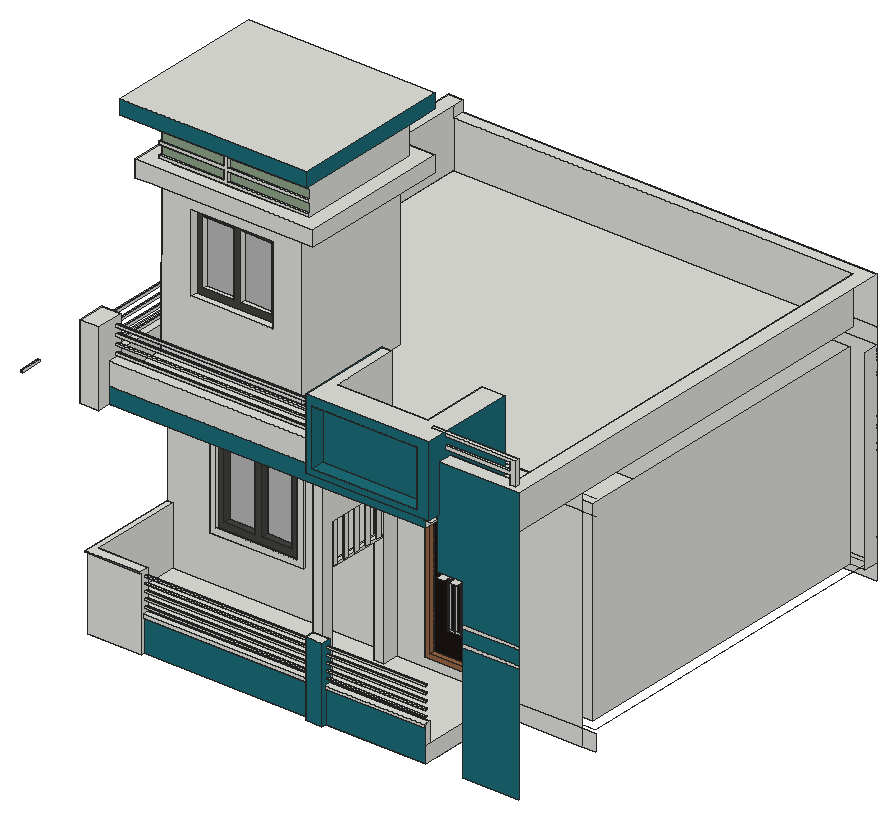
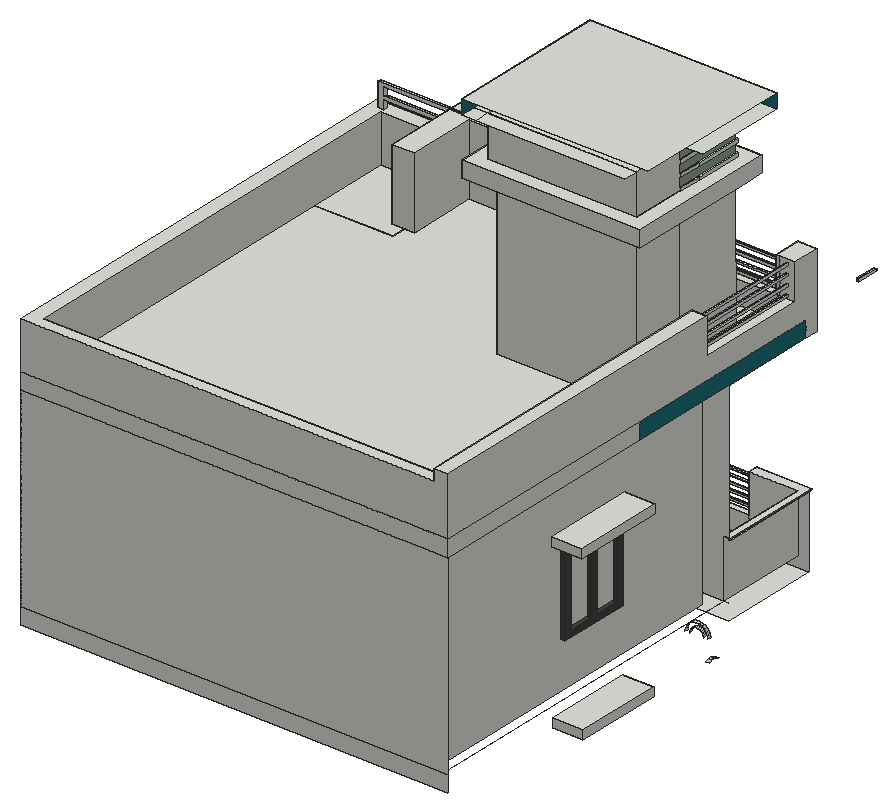
# SketchUp Ruby script. Lengths in inches.
U = 1.inch
M = Sketchup.active_model
def pt(a) = Geom::Point3d.new(a.map { |v| v * U })
def face(e, loops, mat)
  f = e.add_face(loops[0].map { |a| pt(a) })
  loops[1..].each { |l| e.add_face(l.map { |a| pt(a) }).erase! }
  f.material = f.back_material = mat if mat
  f
end
# faces: each face lists its corners as indices into pts; further lists are holes
def faces(e, pts, list, mat = nil) = list.each { |f| face(e, (f[0].is_a?(Array) ? f : [f]).map { |l| l.map { |i| pts[i] } }, mat) }
# xy, xz, yz: faces in a plane at the given z, y or x. An outline is a flat list of corners, or four numbers for a rectangle; further outlines are holes
def ring(l) = l.size == 4 ? [[l[0], l[1]], [l[2], l[1]], [l[2], l[3]], [l[0], l[3]]] : l.each_slice(2).to_a
def flat(e, list, mat, &to3) = list.each { |f| face(e, (f[0].is_a?(Array) ? f : [f]).map { |l| ring(l).map { |u, v| to3.(u, v) } }, mat) }
def xy(e, z, list, mat = nil) = flat(e, list, mat) { |x, y| [x, y, z] }
def xz(e, y, list, mat = nil) = flat(e, list, mat) { |x, z| [x, y, z] }
def yz(e, x, list, mat = nil) = flat(e, list, mat) { |y, z| [x, y, z] }
def lines(e, pts, list) = list.each { |a, b| e.add_line(pt(pts[a]), pt(pts[b])) }
# prism: a flat outline (further loops are holes) pulled along v
def prism(e, loops, v, mat = nil)
  f = face(e, loops, mat); d = Geom::Vector3d.new(v.map { |x| x * U })
  f.pushpull(f.normal.samedirection?(d) ? d.length : -d.length)
end
def box(e, o, s, mat = nil) = prism(e, [[o, [o[0] + s[0], o[1], o[2]], [o[0] + s[0], o[1] + s[1], o[2]], [o[0], o[1] + s[1], o[2]]]], [0, 0, s[2]], mat)
def at(x, y, z, deg = 0) = Geom::Transformation.translation(pt([x, y, z])) * Geom::Transformation.rotation(ORIGIN, Z_AXIS, deg.degrees)
def axes(o, x, y, z) = Geom::Transformation.new([*x, 0, *y, 0, *z, 0, *pt(o).to_a, 1])
def part(name) = M.definitions.add(name)
# library, detail: a bought-in or finely detailed component or shape, given as its bounding box
def library(name, o, s) = part(name).tap { |d| box(d.entities, o, s) }
def detail(e, o, s) = box(e.add_group.entities, o, s)
def put(e, d, t, mat = nil) = e.add_instance(d, t).tap { |i| i.material = mat if mat }
def group(e, t, mat = nil) = e.add_group.tap { |g| g.transformation = t; g.material = mat if mat }.entities
root = M.entities
M.materials.add("Glass_Mirror_01").color = [185, 185, 185]
M.materials.add("I06_Sapphire_Night").color = [28, 110, 122]
M.materials.add("M04_Stone_Frost").color = [142, 163, 138]
M.materials.add("M05_Graphite_Haze").color = [114, 114, 114]
M.materials.add("Wood_Floor_12_1K").color = [28, 22, 19]
M.materials.add("Wood_Planks_01_1K").color = [69, 67, 63]
M.materials.add("Wood_Veneer_15_1K").color = [153, 102, 66]
box(root,[5.27,10.71,299.4],[1.43,13.32,1.36])
xy(root,139.3,[[15.64,197.5,18.64,213.54],[15.64,217.54,18.64,233.59]],"Wood_Planks_01_1K")
xy(root,143.3,[[15.64,193.5,18.64,237.59]])
xy(root,144,[[153.64,45,153.64,48,51.78,48,51.78,46,18.64,46,18.64,108,153.64,108,153.64,50.875,159.64,50.875,159.64,56.88,225.64,56.88,225.64,108,225.72,108,225.72,48,164.1,48,164.1,45],[153.64,50.875,153.64,108,225.64,108,225.64,56.88,159.64,56.88,159.64,50.875],[153.64,50.875,159.64,108],[159.64,56.88,225.64,108]])
xy(root,144.51,[[0,189.1,18.64,243.39]])
xy(root,149.79,[[0,189.1,18.64,243.39]])
xy(root,154,[[225.64,48,225.72,48,225.72,108,159.64,108,159.64,98,153.64,98,153.64,108,21.64,108,21.64,51,153.64,51,153.64,58,159.64,58,159.64,51,225.64,51],[153.64,50.875,159.64,51],[153.64,51,159.64,58],[27.64,117,273.64,315]])
xy(root,160,[[177.64,108,213.64,117]])
xy(root,160,[[177.64,107,213.64,108]],"Wood_Veneer_15_1K")
xy(root,163,[[180.64,110.5,210.64,117]])
xy(root,163,[[180.64,107,210.64,110.5]],"Wood_Veneer_15_1K")
xy(root,164,[[51.78,47,153.64,48],[164.1,47,225.64,48]])
xy(root,166,[[51.78,47,153.64,47,153.64,50.875,164.1,50.875,164.1,47,225.64,47,225.64,51,51.78,51]])
xy(root,169.1,[[51.78,47.89,225.64,49.04]])
xy(root,170.1,[[51.78,47.89,225.64,49.04]])
xy(root,173.43,[[51.78,47.89,225.64,49.04]])
xy(root,174.42,[[51.78,47.89,225.64,49.04]])
xy(root,177.74,[[190.19,109.5,202.59,110.5]])
xy(root,177.75,[[51.78,47.89,225.64,49.04]])
xy(root,178.74,[[51.78,47.89,225.64,49.04],[191.19,109.5,193.99,110.5],[194.99,109.5,197.79,110.5],[198.79,109.5,201.59,110.5]])
xy(root,182.08,[[51.78,47.89,225.64,49.04]])
xy(root,182.6,[[45.44,106.82,103.01,108]])
xy(root,183.07,[[51.78,47.89,225.64,49.04]])
xy(root,186.4,[[51.78,47.89,225.64,49.04],[49.24,106.82,99.21,108]])
xy(root,187.39,[[51.78,47.89,225.64,49.04]])
xy(root,189,[[17.64,45,50.78,46],[50.78,45,51.78,46],[17.64,46,18.64,107],[17.64,107,18.64,108]])
xy(root,190,[[17.64,45,51.78,45,51.78,51,21.64,51,21.64,108,17.64,108],[153.64,45,164.1,50.875]])
xy(root,190.4,[[53.24,112.5,72.22,117],[76.22,112.5,95.21,117]])
xy(root,190.4,[[53.24,108,72.22,112.5],[76.22,108,95.21,112.5]],"Wood_Planks_01_1K")
xy(root,190.875,[[15.64,193.5,18.64,237.59]],"Wood_Planks_01_1K")
xy(root,194.875,[[15.64,197.5,18.64,213.54],[15.64,217.54,18.64,233.59]],"Wood_Planks_01_1K")
xy(root,205.66,[[191.19,109.5,193.99,110.5],[194.99,109.5,197.79,110.5],[198.79,109.5,201.59,110.5]])
xy(root,206.43,[[191.19,109.5,193.99,110.5],[194.99,109.5,197.79,110.5],[198.79,109.5,201.59,110.5]])
xy(root,223.3125,[[155.41,58,158.36,98]])
xy(root,224.34,[[191.19,109.5,193.99,110.5],[194.99,109.5,197.79,110.5],[198.79,109.5,201.59,110.5]])
xy(root,224.66,[[155.41,58,158.36,58,158.36,59.95,158.14,59.95,158.14,62.61,158.36,62.61,158.36,68.33,158.14,68.33,158.14,70.98,158.36,70.98,158.36,76.7,158.14,76.7,158.14,79.36,158.36,79.36,158.36,85.08,158.14,85.08,158.14,87.73,158.36,87.73,158.36,93.45,158.14,93.45,158.14,96.11,158.36,96.11,158.36,98,155.41,98],[158.14,59.95,158.36,62.61],[158.36,59.95,159.05,62.61],[158.14,68.33,158.36,70.98],[158.36,68.33,159.05,70.98],
  [158.14,76.7,158.36,79.36],[158.36,76.7,159.05,79.36],[158.14,85.08,158.36,87.73],[158.36,85.08,159.05,87.73],[158.14,93.45,158.36,96.11],
  [158.36,93.45,159.05,96.11]])
xy(root,225.34,[[190.19,109.5,202.59,110.5]])
xy(root,237.72,[[53.24,112.5,72.22,117],[76.22,112.5,95.21,117]])
xy(root,237.72,[[53.24,108,72.22,112.5],[76.22,108,95.21,112.5]],"Wood_Planks_01_1K")
xy(root,237.76,[[15.64,197.5,18.64,213.54],[15.64,217.54,18.64,233.59]],"Wood_Planks_01_1K")
xy(root,241,[[180.64,110.5,210.64,117]])
xy(root,241,[[180.64,107,210.64,110.5]],"Wood_Veneer_15_1K")
xy(root,241.72,[[49.24,106.82,99.21,108]])
xy(root,241.76,[[15.64,193.5,18.64,237.59]],"Wood_Planks_01_1K")
xy(root,244,[[177.64,108,213.64,117]])
xy(root,244,[[177.64,107,213.64,108]],"Wood_Veneer_15_1K")
xy(root,244.92,[[0,187.98,18.64,244.27]])
xy(root,245.52,[[45.44,106.82,103.01,108]])
xy(root,250,[[[153.64,58,159.64,98],[158.14,85.08,159.05,87.73],[158.14,76.7,159.05,79.36],[158.14,68.33,159.05,70.98],[158.14,59.95,159.05,62.61],[158.14,93.45,159.05,96.11]],[158.14,59.95,159.05,62.61],[158.14,68.33,159.05,70.98],[158.14,76.7,159.05,79.36],[158.14,85.08,159.05,87.73],
  [158.14,93.45,159.05,96.11]])
xy(root,250.47,[[0,187.98,18.64,244.27]])
xy(root,252.41,[[236.45,43,240.8,48],[244.33,43,248.68,48]])
xy(root,274,[[18.64,40,30.27,48],[18.64,48,18.64,108,153.64,108,153.64,50.875,159.64,50.875,159.64,108,225.72,108,225.72,48]])
xy(root,281.97,[[228.57,43,232.92,48]])
xy(root,284,[[18.64,48,225.72,48,225.72,57,225.64,57,225.64,108,273.64,108,273.64,317.1,27.64,317.1,27.64,324,18.64,324],[225.64,57,225.72,108],[225.72,57,273.64,108]])
xy(root,284.16,[[18.64,48,18.64,324,27.64,324,27.64,57,157.87,57,157.87,98.875,163.87,98.875,163.87,57,219.64,57,219.64,98.875,233.62,98.875,233.62,57,225.64,57,225.64,48]])
xy(root,284.16,[[157.87,40,233.62,48]],"I06_Sapphire_Night")
xy(root,288.16,[[161.87,40,226.3,48]],"I06_Sapphire_Night")
xy(root,298.07,[[30.27,48,157.87,57],[18.64,57,27.64,124.99]])
xy(root,299.02,[[22.93,57,24.36,121.44],[22.93,121.44,24.36,124.99]])
xy(root,299.4,[[30.27,52.5,157.87,53.93]])
xy(root,300.38,[[22.93,57,24.36,121.44],[22.93,121.44,24.36,124.99]])
xy(root,300.76,[[30.27,52.5,157.87,53.93]])
xy(root,304.59,[[30.27,52.5,157.87,53.93]])
xy(root,304.82,[[22.93,57,24.36,121.44],[22.93,121.44,24.36,124.99]])
xy(root,305.95,[[30.27,52.5,157.87,53.93]])
xy(root,306.18,[[22.93,57,24.36,121.44],[22.93,121.44,24.36,124.99]])
xy(root,309.78,[[30.27,52.5,157.87,53.93]])
xy(root,310.63,[[22.93,57,24.36,121.44],[22.93,121.44,24.36,124.99]])
xy(root,311.14,[[30.27,52.5,157.87,53.93]])
xy(root,311.99,[[22.93,57,24.36,121.44],[22.93,121.44,24.36,124.99]])
xy(root,313.32,[[[233.62,48,282.64,48,282.64,324,27.64,324,27.64,317.1,273.64,317.1,273.64,57,233.62,57],[274.2,52.33,277.71,54.32]],[225.64,48,233.62,57]])
xy(root,314.97,[[30.27,52.5,157.87,53.93]])
xy(root,316.33,[[30.27,52.5,157.87,53.93]])
xy(root,316.43,[[22.93,57,24.36,121.44],[22.93,121.44,24.36,124.99]])
xy(root,317.79,[[22.93,57,24.36,121.44],[22.93,121.44,24.36,124.99]])
xy(root,318.66,[[225.69,52.33,274.2,54.32]])
xy(root,320,[[18.64,40,30.27,57],[18.64,124.99,27.64,324]])
xy(root,320.03,[[45.8,91.34,96.39,95.875]])
xy(root,320.71,[[225.69,52.33,274.2,54.32]])
xy(root,322.89,[[161.87,40,226.3,48]])
xy(root,324.03,[[49.8,95.875,69.1,98.875],[73.1,95.875,92.39,98.875]])
xy(root,325.78,[[225.69,52.33,274.2,54.32]])
xy(root,327.87,[[157.87,40,233.62,40,233.62,52.33,225.69,52.33,225.69,54.32,233.62,54.32,233.62,98.875,219.64,98.875,219.64,57,163.87,57,163.87,98.875,157.87,98.875],[225.69,52.33,233.62,54.32],[233.62,52.33,277.71,54.32]])
xy(root,364.13,[[49.8,95.875,69.1,98.875],[73.1,95.875,92.39,98.875]])
xy(root,368.13,[[45.8,91.34,96.39,95.875]])
xy(root,380.13,[[27.82,82.27,114.51,91.34],[27.82,91.34,114.51,167.15],[27.82,167.15,114.51,176.22]])
xy(root,390.13,[[27.84,90.34,67.09,91.34],[67.09,90.34,69.71,91.34],[69.71,90.34,119.53,91.34],[26.84,120.18,27.84,134.17]])
xy(root,392.13,[[26.84,90.34,27.84,120.18],[27.84,90.34,67.09,91.34],[69.71,90.34,119.53,91.34],[26.84,120.18,27.84,134.17]])
xy(root,397.81,[[26.85,90.34,27.85,120.18],[27.85,90.34,67.1,91.34],[69.72,90.34,119.54,91.34],[26.85,120.18,27.85,134.17]])
xy(root,399.81,[[26.86,90.34,27.86,120.18],[27.86,90.34,67.1,91.34],[69.72,90.34,119.55,91.34],[26.86,120.18,27.86,134.17]])
xy(root,405.49,[[26.87,90.34,27.87,120.18],[27.87,90.34,67.12,91.34],[69.73,90.34,119.56,91.34],[26.87,120.18,27.87,134.17]])
xy(root,407.49,[[26.875,90.34,27.875,120.18],[27.875,90.34,67.12,91.34],[69.74,90.34,119.56,91.34],[26.875,120.18,27.875,134.17]])
xy(root,413.16,[[27.88,90.34,67.13,91.34],[69.75,90.34,119.57,91.34]])
xy(root,415.16,[[27.89,77.1875,119.58,90.34],[27.89,90.34,119.58,167.15],[27.89,167.15,119.58,176.1875]])
xz(root,40,[[18.64,274,30.27,320]])
xz(root,40,[[[157.87,284.16,233.62,327.87],[161.87,288.16,226.3,322.89]]],"I06_Sapphire_Night")
xz(root,45,[[153.64,144,164.1,190]],"I06_Sapphire_Night")
xz(root,45,[[17.64,189,51.78,190]],"M05_Graphite_Haze")
xz(root,46,[[18.64,144,51.78,189]])
xz(root,47,[[51.78,164,153.64,166],[164.1,164,225.64,166]])
xz(root,47.89,[[51.78,169.1,225.64,170.1],[51.78,173.43,225.64,174.42],[51.78,177.75,225.64,178.74],[51.78,182.08,225.64,183.07],[51.78,186.4,225.64,187.39]])
xz(root,48,[[225.64,144,225.72,154],[248.68,216.18,282.64,218.18],[248.68,226.69,282.64,228.69],[18.64,274,30.27,284],[225.64,274,225.72,284],
  [18.64,284,30.27,284.16],[157.87,284,225.64,284.16],[225.64,284,225.72,284,232.92,284.15,232.92,284.16,225.64,284.16],[232.92,284.15,233.62,284.16,232.92,284.16],[30.27,284.16,157.87,298.07],
  [225.64,284.16,233.62,284.16,233.62,313.32,226.3,313.32,226.3,288.16,225.64,288.16]])
xz(root,48,[[51.78,144,153.64,164],[164.1,144,225.64,164],[248.68,144,282.64,216.18],[248.68,218.18,282.64,226.69],[248.68,228.69,282.64,228.69,282.64,313.32,233.62,313.32,233.62,284.16,232.92,284.15,232.92,252.41,248.68,252.41],
  [30.27,274,225.64,284],[161.87,288.16,226.3,322.89]],"I06_Sapphire_Night")
xz(root,49.04,[[51.78,169.1,225.64,170.1],[51.78,173.43,225.64,174.42],[51.78,177.75,225.64,178.74],[51.78,182.08,225.64,183.07],[51.78,186.4,225.64,187.39]])
xz(root,50.875,[[153.64,154,159.64,166],[153.64,166,159.64,190],[159.64,166,164.1,190],[153.64,190,159.64,274]])
xz(root,51,[[21.64,154,51.78,190],[51.78,154,225.64,166]])
xz(root,52.33,[[274.2,313.32,277.71,313.32,277.71,327.87,225.69,327.87,225.69,325.78,274.2,325.78,274.2,320.71,225.69,320.71,225.69,318.66,274.2,318.66]])
xz(root,52.5,[[30.27,299.4,157.87,300.76],[30.27,304.59,157.87,305.95],[30.27,309.78,157.87,311.14],[30.27,314.97,157.87,316.33]])
xz(root,53.93,[[30.27,299.4,157.87,300.76],[30.27,304.59,157.87,305.95],[30.27,309.78,157.87,311.14],[30.27,314.97,157.87,316.33]])
xz(root,54.32,[[274.2,313.32,274.2,318.66,225.69,318.66,225.69,320.71,274.2,320.71,274.2,325.78,225.69,325.78,225.69,327.87,277.71,327.87,277.71,313.32]])
xz(root,57,[[225.64,284,225.64,284.16,233.62,284.16,233.62,313.32,273.64,313.32,273.64,284],[27.64,284.16,157.87,298.07],[163.87,284.16,219.64,327.87],[225.64,284.16,233.62,313.32],[[18.64,298.07,27.64,320],[22.93,316.43,24.36,317.79],[22.93,304.82,24.36,306.18],[22.93,299.02,24.36,300.38],[22.93,310.63,24.36,311.99]],
  [27.64,298.07,30.27,320]])
xz(root,58,[[[153.64,154,159.64,250],[155.41,223.3125,158.36,224.66]],[155.41,223.3125,158.36,224.66]])
xz(root,59.95,[[158.14,224.66,159.05,250]])
xz(root,62.61,[[158.14,224.66,159.05,250]])
xz(root,68.33,[[158.14,224.66,159.05,250]])
xz(root,70.98,[[158.14,224.66,159.05,250]])
xz(root,76.7,[[158.14,224.66,159.05,250]])
xz(root,77.1875,[[128.58,415.15,128.6,423.97,13.75,424.19,13.74,415.19,27.89,415.16,119.58,415.16]],"I06_Sapphire_Night")
xz(root,79.36,[[158.14,224.66,159.05,250]])
xz(root,82.27,[[128.58,380.1,128.59,389.9375,18.77,390.15,18.75,380.15,27.82,380.13,114.51,380.13]])
xz(root,85.08,[[158.14,224.66,159.05,250]])
xz(root,87.73,[[158.14,224.66,159.05,250]])
xz(root,90.34,[[26.84,390.13,119.53,390.13,119.53,392.13,69.71,392.13,69.72,397.81,119.54,397.81,119.55,399.81,69.72,399.81,69.73,405.49,119.56,405.49,119.56,407.49,69.74,407.49,69.75,413.16,119.57,413.16,119.58,415.16,27.89,415.16,26.89,415.17,26.88,413.17,27.88,413.16,67.13,413.16,67.12,407.49,26.875,407.49,26.87,405.49,67.12,405.49,67.1,399.81,26.86,399.81,26.85,397.81,67.1,397.81,67.09,392.13,26.84,392.13]])
xz(root,91.34,[[[114.33,284,114.51,380.13,27.82,380.13,27.64,284.36,27.64,284.16],[45.8,320.03,96.39,368.13]],[119.53,389.96,119.53,390.13,69.71,390.13,69.71,390.05,114.53,389.97],[69.71,390.05,69.71,390.13,67.09,390.13,67.09,390.06],[67.09,390.06,67.09,390.13,27.84,390.13]])
xz(root,91.34,[[27.84,392.13,67.09,392.13,67.1,397.81,27.85,397.81],[69.71,392.13,119.53,392.13,119.54,397.81,69.72,397.81],[27.86,399.81,67.1,399.81,67.12,405.49,27.87,405.49],[69.72,399.81,119.55,399.81,119.56,405.49,69.73,405.49],[27.875,407.49,67.12,407.49,67.13,413.16,27.88,413.16,27.88,411.16],
  [69.74,407.49,119.56,407.49,119.57,413.16,69.75,413.16]],"M04_Stone_Frost")
xz(root,93.45,[[158.14,224.66,159.05,250]])
xz(root,95.875,[[[45.8,320.03,96.39,368.13],[49.8,324.03,69.1,364.13],[73.1,324.03,92.39,364.13]]],"Wood_Planks_01_1K")
xz(root,96.11,[[158.14,224.66,159.05,250]])
xz(root,98,[[[153.64,154,159.64,250],[155.41,223.3125,158.36,224.66]],[155.41,223.3125,158.36,224.66]])
xz(root,98.875,[[157.87,284.16,163.87,327.87],[219.64,284.16,233.62,327.87]])
xz(root,98.875,[[49.8,324.03,69.1,364.13],[73.1,324.03,92.39,364.13]],"Glass_Mirror_01")
xz(root,106.82,[[[45.44,182.6,103.01,245.52],[49.24,186.4,99.21,241.72]]])
xz(root,107,[[[177.64,160,213.64,244],[180.64,163,210.64,241]]],"Wood_Veneer_15_1K")
xz(root,108,[[225.64,144,225.72,154],[225.72,144,231.64,154],[231.64,144,273.64,154],[273.64,144,282.64,154],[[21.64,154,153.64,154,153.64,274,18.64,274,18.64,190,21.64,190],[45.44,182.6,103.01,245.52]],
  [[159.64,154,225.64,274],[177.64,160,213.64,244]],[225.64,154,231.64,274],[231.64,154,273.64,274],[225.64,274,225.72,284],[225.72,274,231.64,284],
  [231.64,274,273.64,284]])
xz(root,108,[[17.64,189,18.64,190]],"M05_Graphite_Haze")
xz(root,108,[[[49.24,186.4,99.21,241.72],[53.24,190.4,72.22,237.72],[76.22,190.4,95.21,237.72]]],"Wood_Planks_01_1K")
xz(root,109.5,[[[190.19,177.74,202.59,225.34],[198.79,178.74,198.79,205.66,201.59,205.66,201.59,206.43,198.79,206.43,198.79,224.34,201.59,224.34,201.59,178.74],[194.99,178.74,197.79,205.66],[191.19,178.74,193.99,205.66],[194.99,206.43,197.79,224.34],[191.19,206.43,193.99,224.34]]])
xz(root,110.5,[[[180.64,163,210.64,241],[190.19,177.74,202.59,225.34]],[191.19,178.74,193.99,205.66],[194.99,178.74,197.79,205.66],[198.79,178.74,201.59,205.66],[191.19,206.43,193.99,224.34],
  [194.99,206.43,197.79,224.34],[198.79,206.43,201.59,224.34]],"Wood_Floor_12_1K")
xz(root,112.5,[[53.24,190.4,72.22,237.72],[76.22,190.4,95.21,237.72]],"Glass_Mirror_01")
xz(root,117,[[[27.64,154,273.64,274],[177.64,160,213.64,244],[53.24,190.4,72.22,237.72],[76.22,190.4,95.21,237.72]]])
xz(root,120.18,[[26.84,390.13,27.84,392.13],[26.85,397.81,27.85,397.81,27.86,399.81,26.86,399.81],[26.87,405.49,27.87,405.49,27.875,407.49,26.875,407.49],[27.88,413.16,27.89,415.16,26.89,415.17,26.88,413.17]])
xz(root,121.44,[[22.93,299.02,24.36,300.38],[22.93,304.82,24.36,306.18],[22.93,310.63,24.36,311.99],[22.93,316.43,24.36,317.79]])
xz(root,124.99,[[[18.64,298.07,27.64,320],[22.93,299.02,24.36,300.38],[22.93,304.82,24.36,306.18],[22.93,310.63,24.36,311.99],[22.93,316.43,24.36,317.79]]])
xz(root,157.4,[[177.64,160,213.64,244]])
xz(root,167.15,[[114.33,284,27.64,284.16,27.64,284.36,27.82,380.13,114.51,380.13],[119.53,389.96,27.84,390.13,27.89,415.16,119.58,415.16]])
xz(root,176.22,[[128.58,380.1,114.51,380.13,27.82,380.13,18.75,380.15,18.77,390.15,27.84,390.13,128.59,389.9375]])
xz(root,187.98,[[0,244.92,18.64,250.47]])
xz(root,189.1,[[0,144.51,18.64,149.79]])
xz(root,193.5,[[15.64,190.875,18.64,241.76]])
xz(root,197.5,[[15.64,194.875,18.64,237.76]],"Wood_Planks_01_1K")
xz(root,213.54,[[15.64,194.875,18.64,237.76]])
xz(root,217.54,[[15.64,194.875,18.64,237.76]],"Wood_Planks_01_1K")
xz(root,233.59,[[15.64,194.875,18.64,237.76]])
xz(root,237.59,[[15.64,190.875,18.64,241.76]],"Wood_Planks_01_1K")
xz(root,243.39,[[0,144.51,18.64,149.79]])
xz(root,244.27,[[0,244.92,18.64,250.47]])
xz(root,315,[[27.64,154,273.64,274]])
xz(root,317.1,[[27.64,284,273.64,313.32]])
xz(root,324,[[18.64,144,282.64,154],[18.64,154,282.64,274],[18.64,274,282.64,284],[27.64,284,27.64,284.16,18.64,284.16,18.64,320,27.64,320,27.64,313.32,282.64,313.32,282.64,284]])
yz(root,0,[[189.1,144.51,243.39,149.79],[187.98,244.92,244.27,250.47]])
yz(root,15.64,[[[193.5,190.875,237.59,241.76],[217.54,194.875,233.59,237.76],[197.5,194.875,213.54,237.76]]],"Wood_Planks_01_1K")
yz(root,17.64,[[45,189,108,190]],"M05_Graphite_Haze")
yz(root,18.64,[[197.5,194.875,213.54,237.76],[217.54,194.875,233.59,237.76],[40,274,40,320,57,320,57,298.07,124.99,298.07,124.99,320,324,320,324,284.16,48,284.16,48,274],[176.54,274,324,284]])
yz(root,18.64,[[48,274,176.54,284]],"I06_Sapphire_Night")
yz(root,21.64,[[51,154,108,190]])
yz(root,22.93,[[57,299.02,121.44,300.38],[121.44,299.02,124.99,300.38],[57,304.82,121.44,306.18],[121.44,304.82,124.99,306.18],[57,310.63,121.44,311.99],
  [121.44,310.63,124.99,311.99],[57,316.43,121.44,317.79],[121.44,316.43,124.99,317.79]])
yz(root,24.36,[[57,299.02,121.44,300.38],[121.44,299.02,124.99,300.38],[57,304.82,121.44,306.18],[121.44,304.82,124.99,306.18],[57,310.63,121.44,311.99],
  [121.44,310.63,124.99,311.99],[57,316.43,121.44,317.79],[121.44,316.43,124.99,317.79]])
yz(root,26.84,[[90.34,390.13,120.18,392.13],[120.18,390.13,134.17,392.13]])
yz(root,27.64,[[117,154,315,274],[317.1,284,324,284.16],[57,284.16,91.34,284.16,91.34,284.36,167.15,284.36,167.15,284.16,317.1,284.16,317.1,320,124.99,320,124.99,298.07,57,298.07],[91.34,284.16,134.17,284.36],[134.17,284.16,167.15,284.36],
  [134.17,284.16,167.15,284.36],[317.1,313.32,324,320]])
yz(root,30.27,[[[40,274,48,274,48,298.07,57,298.07,57,320,40,320],[52.5,314.97,53.93,316.33],[52.5,309.78,53.93,311.14],[52.5,304.59,53.93,305.95],[52.5,299.4,53.93,300.76]]])
yz(root,45.44,[[106.82,182.6,108,245.52]])
yz(root,45.8,[[91.34,320.03,95.875,368.13]])
yz(root,49.24,[[106.82,186.4,108,241.72]])
yz(root,49.8,[[95.875,324.03,98.875,364.13]])
yz(root,51.78,[[[46,144,46,189,45,189,45,190,51,190,51,166,47,166,47,164,48,164,48,144],[47.89,186.4,49.04,187.39],[47.89,182.08,49.04,183.07],[47.89,177.75,49.04,178.74],[47.89,173.43,49.04,174.42],[47.89,169.1,49.04,170.1]],[47.89,169.1,49.04,170.1],[47.89,173.43,49.04,174.42],[47.89,177.75,49.04,178.74],[47.89,182.08,49.04,183.07],
  [47.89,186.4,49.04,187.39]])
yz(root,53.24,[[112.5,190.4,117,237.72]])
yz(root,53.24,[[108,190.4,112.5,237.72]],"Wood_Planks_01_1K")
yz(root,69.1,[[95.875,324.03,98.875,364.13]])
yz(root,72.22,[[112.5,190.4,117,237.72]])
yz(root,72.22,[[108,190.4,112.5,237.72]],"Wood_Planks_01_1K")
yz(root,73.1,[[95.875,324.03,98.875,364.13]])
yz(root,76.22,[[112.5,190.4,117,237.72]])
yz(root,76.22,[[108,190.4,112.5,237.72]],"Wood_Planks_01_1K")
yz(root,92.39,[[95.875,324.03,98.875,364.13]])
yz(root,95.21,[[112.5,190.4,117,237.72]])
yz(root,95.21,[[108,190.4,112.5,237.72]],"Wood_Planks_01_1K")
yz(root,96.39,[[91.34,320.03,95.875,368.13]])
yz(root,99.21,[[106.82,186.4,108,241.72]])
yz(root,103.01,[[106.82,182.6,108,245.52]])
yz(root,153.64,[[50.875,154,50.875,274,108,274,108,154,98,154,98,250,58,250,58,154]])
yz(root,153.64,[[45,144,45,190,50.875,190,50.875,166,47,166,47,164,48,164,48,144]],"I06_Sapphire_Night")
yz(root,155.41,[[58,223.3125,98,224.66]])
yz(root,157.87,[[[40,284.16,40,327.87,98.875,327.87,98.875,284.16,57,284.16,57,298.07,48,298.07,48,284.16],[52.5,314.97,53.93,316.33],[52.5,309.78,53.93,311.14],[52.5,304.59,53.93,305.95],[52.5,299.4,53.93,300.76]]],"I06_Sapphire_Night")
yz(root,158.14,[[59.95,224.66,62.61,250],[68.33,224.66,70.98,250],[76.7,224.66,79.36,250],[85.08,224.66,87.73,250],[93.45,224.66,96.11,250]])
yz(root,158.36,[[58,223.3125,98,224.66]])
yz(root,159.05,[[59.95,224.66,62.61,250],[68.33,224.66,70.98,250],[76.7,224.66,79.36,250],[85.08,224.66,87.73,250],[93.45,224.66,96.11,250]])
yz(root,159.64,[[50.875,154,58,154,58,250,98,250,98,154,108,154,108,274,50.875,274]])
yz(root,161.87,[[40,288.16,48,322.89]],"I06_Sapphire_Night")
yz(root,163.87,[[57,284.16,98.875,327.87]])
yz(root,164.1,[[45,144,48,144,48,164,47,164,47,166,50.875,166,50.875,190,45,190]],"I06_Sapphire_Night")
yz(root,177.64,[[108,160,117,244]])
yz(root,177.64,[[107,160,108,244]],"Wood_Veneer_15_1K")
yz(root,180.64,[[110.5,163,117,241]])
yz(root,180.64,[[107,163,110.5,241]],"Wood_Veneer_15_1K")
yz(root,190.19,[[109.5,177.74,110.5,225.34]])
yz(root,191.19,[[109.5,178.74,110.5,205.66],[109.5,206.43,110.5,224.34]])
yz(root,193.99,[[109.5,178.74,110.5,205.66],[109.5,206.43,110.5,224.34]])
yz(root,194.99,[[109.5,178.74,110.5,205.66],[109.5,206.43,110.5,224.34]])
yz(root,197.79,[[109.5,178.74,110.5,205.66],[109.5,206.43,110.5,224.34]])
yz(root,198.79,[[109.5,178.74,110.5,205.66],[109.5,206.43,110.5,224.34]])
yz(root,201.59,[[109.5,178.74,110.5,205.66],[109.5,205.66,110.5,206.43],[109.5,206.43,110.5,224.34]])
yz(root,202.59,[[109.5,177.74,110.5,178.74],[109.5,178.74,110.5,224.34],[109.5,224.34,110.5,225.34]])
yz(root,210.64,[[110.5,163,117,241]])
yz(root,210.64,[[107,163,110.5,241]],"Wood_Veneer_15_1K")
yz(root,213.64,[[108,160,117,244]])
yz(root,213.64,[[107,160,108,244]],"Wood_Veneer_15_1K")
yz(root,219.64,[[57,284.16,98.875,327.87]])
yz(root,225.64,[[48,154,51,166],[47,164,48,166],[47.89,169.1,48,170.1],[48,169.1,49.04,170.1],[47.89,173.43,48,174.42],
  [48,173.43,49.04,174.42],[47.89,177.75,48,178.74],[48,177.75,49.04,178.74],[47.89,182.08,48,183.07],[48,182.08,49.04,183.07],
  [47.89,186.4,48,187.39],[48,186.4,49.04,187.39]])
yz(root,225.69,[[52.33,318.66,54.32,320.71],[52.33,325.78,54.32,327.87]])
yz(root,225.72,[[48,144,108,154],[48,274,108,284]])
yz(root,226.3,[[40,288.16,48,322.89]],"I06_Sapphire_Night")
yz(root,233.62,[[40,284.16,48,284.16,48,313.32,57,313.32,57,284.16,98.875,284.16,98.875,327.87,40,327.87]],"I06_Sapphire_Night")
yz(root,273.64,[[117,154,315,274],[57,284,317.1,313.32]])
yz(root,274.2,[[52.33,313.32,54.32,318.66],[52.33,320.71,54.32,325.78]])
yz(root,277.71,[[52.33,313.32,54.32,327.87]])
yz(root,282.64,[[315,154,324,274]])
p = [[18.64,118.125,128.92],[18.64,119.79,129.67],[16.64,119.79,129.67],[16.64,118.125,128.92],[45.29,108,129.01],[45.11,108,130.82],
  [45.11,106,130.82],[45.29,106,129.01],[42.47,108,130.21],[42.58,108,129.09],[42.58,106,129.09],[42.47,106,130.21],
  [18.64,123.4,129.79],[18.64,125.11,129.14],[16.64,125.11,129.14],[16.64,123.4,129.79],[34.02,108,129.37],[34.2,108,130.47],
  [34.2,106,130.47],[34.02,106,129.37],[31.61,108,131.25],[31.32,108,129.45],[31.32,106,129.45],[31.61,106,131.25],
  [18.64,121.59,129.97],[16.64,121.59,129.97],[42.08,108,131.25],[42.08,106,131.25],[34.66,108,131.49],[34.66,106,131.49],
  [44.46,108,132.53],[44.46,106,132.53],[32.37,108,132.92],[32.37,106,132.92],[41.43,108,132.16],[41.43,106,132.16],
  [35.37,108,132.36],[35.37,106,132.36],[40.5625,108,132.87],[40.5625,106,132.87],[36.28,108,133.01],[36.28,106,133.01],
  [43.4,108,134.01],[43.4,106,134.01],[33.52,108,134.33],[33.52,106,134.33],[39.54,108,133.33],[39.54,106,133.33],
  [37.33,108,133.4],[37.33,106,133.4],[38.44,108,133.51],[38.44,106,133.51],[41.99,108,135.17],[41.99,106,135.17],
  [35,108,135.39],[35,106,135.39],[40.33,108,135.92],[40.33,106,135.92],[36.71,108,136.04],[36.71,106,136.04],
  [38.53,108,136.22],[38.53,106,136.22],[114.33,91.34,284],[27.64,91.34,284.16],[27.64,134.17,284.16],[27.64,167.15,284.16],
  [114.33,167.15,284],[114.51,167.15,380.13],[114.51,91.34,380.13],[27.82,91.34,380.13],[27.82,134.17,380.13],[27.64,134.17,284.36],
  [27.64,91.34,284.36],[27.64,167.15,284.36],[27.82,167.15,380.13],[27.82,82.27,380.13],[18.75,82.27,380.15],[18.75,91.34,380.15],
  [18.75,176.22,380.15],[18.77,82.27,390.15],[18.77,176.22,390.15],[114.51,82.27,380.13],[128.58,91.34,380.1],[128.58,82.27,380.1],
  [128.58,176.22,380.1],[128.59,176.22,389.9375],[128.59,82.27,389.9375],[27.82,176.22,380.13],[27.82,176.1875,380.13],[114.51,176.22,380.13],
  [27.84,167.15,390.13],[27.84,134.17,390.13],[67.09,91.34,390.06],[27.84,91.34,390.13],[27.84,90.34,390.13],[26.84,90.34,390.13],
  [26.84,120.18,390.13],[26.84,134.17,390.13],[27.84,176.1875,390.13],[27.84,176.22,390.13],[119.53,167.15,389.96],[119.53,91.34,389.96],
  [114.53,91.34,389.97],[69.71,91.34,390.05],[27.84,120.18,390.13],[119.58,167.15,415.16],[119.58,90.34,415.16],[119.57,90.34,413.16],
  [119.57,91.34,413.16],[119.56,91.34,407.49],[119.56,90.34,407.49],[119.56,90.34,405.49],[119.56,91.34,405.49],[119.55,91.34,399.81],
  [119.55,90.34,399.81],[119.54,90.34,397.81],[119.54,91.34,397.81],[119.53,91.34,392.13],[119.53,90.34,392.13],[119.53,90.34,390.13],
  [119.53,91.34,390.13],[27.84,120.18,392.13],[27.84,134.17,392.13],[27.85,134.17,397.81],[27.85,120.18,397.81],[27.86,120.18,399.81],
  [27.86,134.17,399.81],[27.87,134.17,405.49],[27.87,120.18,405.49],[27.875,120.18,407.49],[27.875,134.17,407.49],[27.88,134.17,413.16],
  [27.88,120.18,413.16],[27.89,120.18,415.16],[27.89,167.15,415.16],[67.1,91.34,397.81],[67.09,91.34,392.13],[67.09,90.34,392.13],
  [67.1,90.34,397.81],[69.71,91.34,392.13],[69.72,91.34,397.81],[69.72,90.34,397.81],[69.71,90.34,392.13],[27.85,91.34,397.81],
  [27.84,91.34,392.13],[26.86,120.18,399.81],[26.85,120.18,397.81],[26.85,90.34,397.81],[26.86,90.34,399.81],[26.86,134.17,399.81],
  [26.85,134.17,397.81],[67.12,91.34,405.49],[67.1,91.34,399.81],[67.1,90.34,399.81],[67.12,90.34,405.49],[69.72,91.34,399.81],
  [69.73,91.34,405.49],[69.73,90.34,405.49],[69.72,90.34,399.81],[27.87,91.34,405.49],[27.86,91.34,399.81],[26.875,120.18,407.49],
  [26.87,120.18,405.49],[26.87,90.34,405.49],[26.875,90.34,407.49],[26.875,134.17,407.49],[26.87,134.17,405.49],[67.13,91.34,413.16],
  [67.12,91.34,407.49],[67.12,90.34,407.49],[67.13,90.34,413.16],[69.74,91.34,407.49],[69.75,91.34,413.16],[69.75,90.34,413.16],
  [69.74,90.34,407.49],[27.88,91.34,411.16],[27.88,91.34,413.16],[27.875,91.34,407.49],[27.88,90.34,413.16],[26.88,90.34,413.17],
  [26.88,120.18,413.17],[26.89,120.18,415.17],[26.89,90.34,415.17],[26.88,134.17,413.17],[26.89,134.17,415.17],[128.58,167.15,415.15],
  [128.58,77.1875,415.15],[119.58,77.1875,415.16],[128.6,176.1875,423.97],[128.6,77.1875,423.97],[128.58,176.1875,415.15],[119.58,176.1875,415.16],
  [13.74,77.1875,415.19],[13.74,134.17,415.19],[27.89,90.34,415.16],[27.89,77.1875,415.16],[13.75,176.1875,424.19],[13.75,77.1875,424.19],
  [193.99,110.5,205.66],[193.99,110.5,206.43],[197.79,110.5,205.66],[197.79,110.5,206.43],[177.64,157.4,160],[177.64,122.34,160],
  [177.64,157.4,244],[177.64,122.34,244],[213.64,157.4,160],[213.64,122.34,160],[213.64,157.4,244],[213.64,122.34,244],
  [159.64,50.875,144],[159.64,50.875,154],[153.64,50.875,144],[153.64,50.875,154],[114.51,167.15,390.13],[67.13,91.34,415.09],
  [69.75,91.34,415.08],[273.64,108,284],[282.64,108,284],[34.06,108,129.23],[34.2,108,130.33],[34.625,108,131.35],
  [35.3,108,132.23],[36.18,108,132.91],[37.2,108,133.33],[38.3,108,133.48],[39.4,108,133.33],[40.43,108,132.91],
  [41.3,108,132.23],[41.98,108,131.35],[42.4,108,130.33],[42.55,108,129.23],[21.64,321,154],[21.64,108,154],
  [222.72,111,154],[279.64,111,154],[279.64,315,154],[279.64,321,154],[153.64,48,164],[164.1,48,164],
  [273.64,315,154],[18.64,108,154],[282.64,315,154],[273.64,108,274],[282.64,108,274]]
faces(root,p,[[0,1,2,3],[4,5,6,7],[8,9,10,11],[12,13,14,15],[16,17,18,19],[20,21,22,23],[1,24,25,2],[24,12,15,25],
  [26,8,11,27],[17,28,29,18],[5,30,31,6],[32,20,23,33],[34,26,27,35],[28,36,37,29],[38,34,35,39],[36,40,41,37],
  [30,42,43,31],[44,32,33,45],[46,38,39,47],[40,48,49,41],[50,46,47,51],[48,50,51,49],[42,52,53,43],[54,44,45,55],
  [52,56,57,53],[58,54,55,59],[56,60,61,57],[60,58,59,61],[62,63,64,65,66],[66,67,68,62],[69,70,71,72],[70,71,73,74],
  [69,75,76,77],[78,77,76,79,80],[81,68,82,83],[82,84,85,86,83],[74,70,69,77,78,87,88],[68,67,89,84,82],[74,90,91,70],[92,93,94,95,96,97,91,90,98,99,80,79,86,85,99,98,90,100,101,102,103],
  [100,90,91,104,96,95,94,93,92,103,102,101],[100,105,106,107,108,109,110,111,112,113,114,115,116,117,118,119,120,101],[91,104,121,122,123,124,125,126,127,128,129,130,131,132,133,134,90],[135,136,137,138],[139,140,141,142],[145,146,147,148],[146,145,149,150],[151,152,153,154],
  [155,156,157,158],[161,162,163,164],[162,161,165,166],[167,168,169,170],[171,172,173,174],[132,176,178,179,180],[181,180,179,182],[132,180,183,131],
  [180,181,184,183],[106,105,185,186,187],[105,191,190,185],[192,193,184,181,182,194,195],[133,194,182,181],[196,197,189,188]])
faces(root,p,[[143,124,123,122,121,144],[159,128,127,126,125,160],[175,176,132,131,130,129,177]],"M04_Stone_Frost")
faces(root,p,[[188,189,186,185,190]],"I06_Sapphire_Night")
lines(root,p,[[198,199],[200,201],[202,203],[204,205],[206,207],[208,209],[210,211],[212,213],[214,102],[167,215],[172,216],[217,218],
  [219,220],[220,221],[221,222],[222,223],[223,224],[224,225],[225,226],[226,227],[227,228],[228,229],[229,230],[230,231],
  [232,233],[234,235],[235,236],[237,232],[238,239],[240,236],[241,233],[236,237],[236,242],[243,244]])
